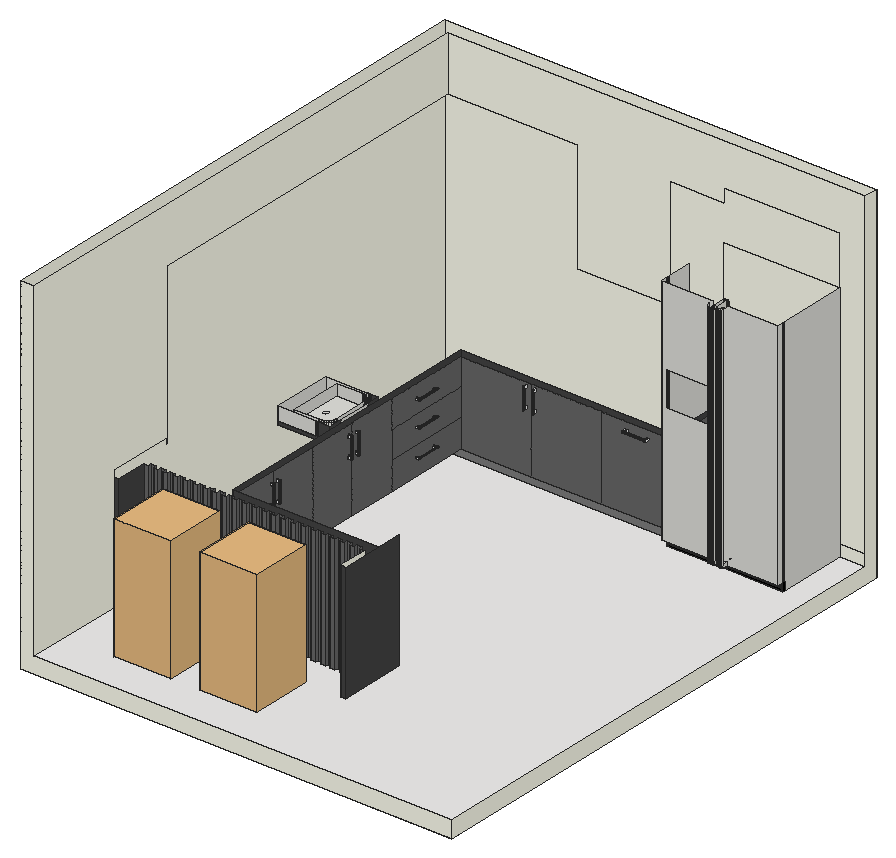
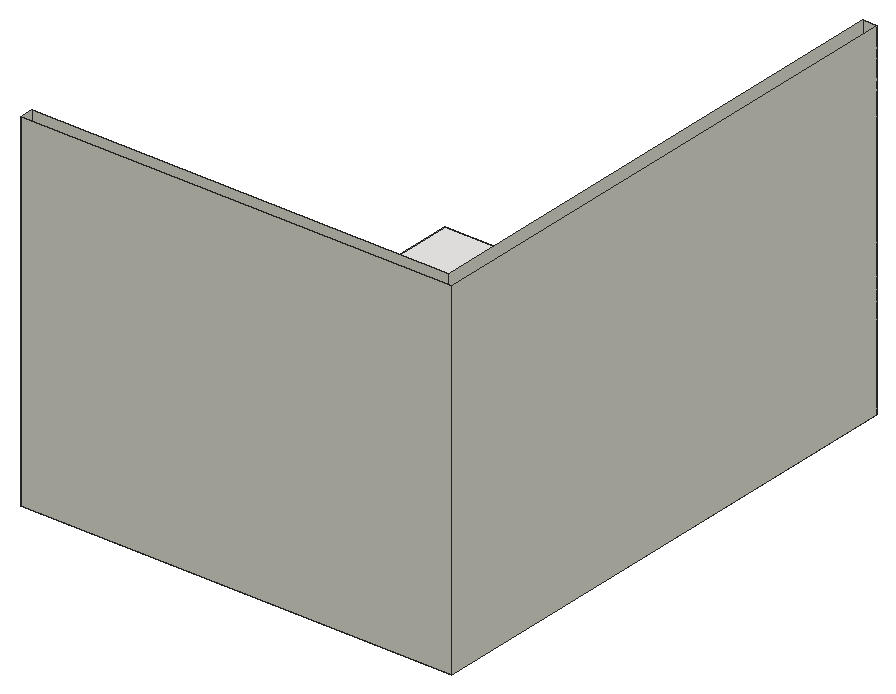
# SketchUp Ruby script. Lengths in inches.
U = 1.inch
M = Sketchup.active_model
def pt(a) = Geom::Point3d.new(a.map { |v| v * U })
def face(e, loops, mat)
  f = e.add_face(loops[0].map { |a| pt(a) })
  loops[1..].each { |l| e.add_face(l.map { |a| pt(a) }).erase! }
  f.material = f.back_material = mat if mat
  f
end
# faces: each face lists its corners as indices into pts; further lists are holes
def faces(e, pts, list, mat = nil) = list.each { |f| face(e, (f[0].is_a?(Array) ? f : [f]).map { |l| l.map { |i| pts[i] } }, mat) }
# xy, xz, yz: faces in a plane at the given z, y or x. An outline is a flat list of corners, or four numbers for a rectangle; further outlines are holes
def ring(l) = l.size == 4 ? [[l[0], l[1]], [l[2], l[1]], [l[2], l[3]], [l[0], l[3]]] : l.each_slice(2).to_a
def flat(e, list, mat, &to3) = list.each { |f| face(e, (f[0].is_a?(Array) ? f : [f]).map { |l| ring(l).map { |u, v| to3.(u, v) } }, mat) }
def xy(e, z, list, mat = nil) = flat(e, list, mat) { |x, y| [x, y, z] }
def xz(e, y, list, mat = nil) = flat(e, list, mat) { |x, z| [x, y, z] }
def yz(e, x, list, mat = nil) = flat(e, list, mat) { |y, z| [x, y, z] }
def lines(e, pts, list) = list.each { |a, b| e.add_line(pt(pts[a]), pt(pts[b])) }
# prism: a flat outline (further loops are holes) pulled along v
def prism(e, loops, v, mat = nil)
  f = face(e, loops, mat); d = Geom::Vector3d.new(v.map { |x| x * U })
  f.pushpull(f.normal.samedirection?(d) ? d.length : -d.length)
end
def box(e, o, s, mat = nil) = prism(e, [[o, [o[0] + s[0], o[1], o[2]], [o[0] + s[0], o[1] + s[1], o[2]], [o[0], o[1] + s[1], o[2]]]], [0, 0, s[2]], mat)
def at(x, y, z, deg = 0) = Geom::Transformation.translation(pt([x, y, z])) * Geom::Transformation.rotation(ORIGIN, Z_AXIS, deg.degrees)
def axes(o, x, y, z) = Geom::Transformation.new([*x, 0, *y, 0, *z, 0, *pt(o).to_a, 1])
def part(name) = M.definitions.add(name)
# library, detail: a bought-in or finely detailed component or shape, given as its bounding box
def library(name, o, s) = part(name).tap { |d| box(d.entities, o, s) }
def detail(e, o, s) = box(e.add_group.entities, o, s)
def put(e, d, t, mat = nil) = e.add_instance(d, t).tap { |i| i.material = mat if mat }
def group(e, t, mat = nil) = e.add_group.tap { |g| g.transformation = t; g.material = mat if mat }.entities
root = M.entities
M.materials.add("[0053_Ivory]").color = [255, 255, 240]
M.materials.add("[0128_White]").color = [255, 255, 255]
M.materials.add("[0133_Gray]").color = [128, 128, 128]
M.materials.add("[0134_DimGray]").color = [105, 105, 105]
M.materials.add("[0137_Black]").color = [0, 0, 0]
M.materials.add("[Granite Dark Gray]").color = [69, 68, 68]
M.materials.add("[Tile Limestone Large]").color = [241, 240, 239]
c1 = library("Group",[-8.82,-17.72,0],[17.64,35.44,18.29])
c2 = part("Bar")
prism(c2.entities,[[[0,0.49,0.31],[0,0.5,0.25],[0,0.49,0.19],[0,0.47,0.125],[0,0.43,0.07],[0,0.375,0.03],[0,0.31,0.01],[0,0.25,0],[0,0.19,0.01],[0,0.125,0.03],[0,0.07,0.07],[0,0.03,0.125],[0,0.01,0.19],[0,0,0.25],[0,0.01,0.31],[0,0.03,0.375],[0,0.07,0.43],[0,0.125,0.47],[0,0.19,0.49],[0,0.25,0.5],[0,0.31,0.49],[0,0.375,0.47],[0,0.43,0.43],[0,0.47,0.375]]],[11.5,0,0],"[0128_White]")
c3 = part("End")
xy(c3.entities,0,[[0,0.25,0.875,1.5]],"[0128_White]")
xy(c3.entities,0.5,[[0,0.25,0.875,1.5]],"[0128_White]")
xz(c3.entities,1.5,[[0,0,0.875,0.5]],"[0128_White]")
yz(c3.entities,0,[[0.25,0,0.19,0.01,0.125,0.03,0.07,0.07,0.03,0.125,0.01,0.19,0,0.25,0.01,0.31,0.03,0.375,0.07,0.43,0.125,0.47,0.19,0.49,0.25,0.5,1.5,0.5,1.5,0]],"[0128_White]")
yz(c3.entities,0.25,[[0.25,0,0.31,0.01,0.375,0.03,0.43,0.07,0.47,0.125,0.49,0.19,0.5,0.25,0.49,0.31,0.47,0.375,0.43,0.43,0.375,0.47,0.31,0.49,0.25,0.5,0.19,0.49,0.125,0.47,0.07,0.43,0.03,0.375,0.01,0.31,0,0.25,0.01,0.19,0.03,0.125,0.07,0.07,0.125,0.03,0.19,0.01]],"[0128_White]")
yz(c3.entities,0.875,[[0.25,0,1.5,0,1.5,0.5,0.25,0.5,0.31,0.49,0.375,0.47,0.43,0.43,0.47,0.375,0.49,0.31,0.5,0.25,0.49,0.19,0.47,0.125,0.43,0.07,0.375,0.03,0.31,0.01]],"[0128_White]")
p = [[0.25,0.125,0.03],[0,0.125,0.03],[0,0.19,0.01],[0.25,0.19,0.01],[0.25,0.07,0.07],[0,0.07,0.07],
  [0,0.25,0],[0.25,0.25,0],[0.875,0.25,0],[0.875,0.31,0.01],[0.25,0.31,0.01],[0.875,0.375,0.03],
  [0.25,0.375,0.03],[0.875,0.43,0.07],[0.25,0.43,0.07],[0.25,0.01,0.19],[0,0.01,0.19],[0,0.03,0.125],
  [0.25,0.03,0.125],[0.875,0.47,0.125],[0.25,0.47,0.125],[0.875,0.49,0.19],[0.25,0.49,0.19],[0.25,0.01,0.31],
  [0,0.01,0.31],[0,0,0.25],[0.25,0,0.25],[0.875,0.5,0.25],[0.25,0.5,0.25],[0.875,0.49,0.31],
  [0.25,0.49,0.31],[0.25,0.03,0.375],[0,0.03,0.375],[0.875,0.47,0.375],[0.25,0.47,0.375],[0.25,0.07,0.43],
  [0,0.07,0.43],[0.25,0.125,0.47],[0,0.125,0.47],[0.875,0.43,0.43],[0.25,0.43,0.43],[0.875,0.375,0.47],
  [0.25,0.375,0.47],[0.25,0.19,0.49],[0,0.19,0.49],[0.25,0.25,0.5],[0,0.25,0.5],[0.875,0.31,0.49],
  [0.875,0.25,0.5],[0.25,0.31,0.49]]
faces(c3.entities,p,[[0,1,2,3],[4,5,1,0],[3,2,6,7],[8,9,10,7],[9,11,12,10],[11,13,14,12],[15,16,17,18],[18,17,5,4],
  [13,19,20,14],[19,21,22,20],[23,24,25,26],[26,25,16,15],[21,27,28,22],[27,29,30,28],[31,32,24,23],[29,33,34,30],
  [35,36,32,31],[37,38,36,35],[33,39,40,34],[39,41,42,40],[43,44,38,37],[45,46,44,43],[47,48,45,49],[41,47,49,42]],"[0128_White]")
c4 = part("Drawer Pull\#1")
put(c4.entities,c2,axes([0.25,0,0],[0.71,0,0],[0,1,0],[0,0,1]))
put(c4.entities,c3,at(0,0,0))
put(c4.entities,c3,axes([8.66,0,0],[-1,0,0],[0,1,0],[0,0,1]),"[0128_White]")
c5 = part("Drawer Pull\#2")
put(c5.entities,c2,axes([0.25,0,0],[0.63,0,0],[0,1,0],[0,0,1]))
put(c5.entities,c3,at(0,0,0))
put(c5.entities,c3,axes([7.74,0,0],[-1,0,0],[0,1,0],[0,0,1]),"[0128_White]")
xy(root,0,[[0,0,156,192]],"[0053_Ivory]")
xy(root,6,[[104.87,161.36,125.37,161.36,125.37,161.85,126.37,161.85,126.37,161.36,146.87,161.36,146.87,187,104.87,187]])
xy(root,6,[[5,0,156,0,156,187,146.87,187,146.87,161.36,126.37,161.36,126.37,161.85,125.37,161.85,125.37,161.36,104.87,161.36,104.87,165,7,165,7,59.91,89,59.91,89,35.93,87,35.93,87,46.93,85.22,46.93,85.22,47.93,83.44,47.93,83.44,46.93,81.67,46.93,81.67,47.93,79.89,47.93,79.89,46.93,78.11,46.93,78.11,47.93,76.33,47.93,76.33,46.93,74.56,46.93,74.56,47.93,72.78,47.93,72.78,46.93,71,46.93,71,47.93,69.22,47.93,69.22,46.93,67.44,46.93,67.44,47.93,65.67,47.93,65.67,46.93,63.89,46.93,63.89,47.93,62.11,47.93,62.11,46.93,60.33,46.93,60.33,47.93,58.56,47.93,58.56,46.93,56.78,46.93,56.78,47.93,55,47.93,55,46.93,53.22,46.93,53.22,47.93,51.44,47.93,51.44,46.93,49.67,46.93,49.67,47.93,47.89,47.93,47.89,46.93,46.11,46.93,46.11,47.93,44.33,47.93,44.33,46.93,42.56,46.93,42.56,47.93,40.78,47.93,40.78,46.93,39,46.93,39,47.93,37.22,47.93,37.22,46.93,35.44,46.93,35.44,47.93,33.67,47.93,33.67,46.93,31.89,46.93,31.89,47.93,30.11,47.93,30.11,46.93,28.33,46.93,28.33,47.93,26.56,47.93,26.56,46.93,24.78,46.93,24.78,47.93,23,47.93,23,46.93,21.22,46.93,21.22,47.93,19.44,47.93,19.44,46.93,17.67,46.93,17.67,47.93,15.89,47.93,15.89,46.93,14.11,46.93,14.11,47.93,12.33,47.93,12.33,46.93,10.56,46.93,10.56,47.93,8.78,47.93,8.78,46.93,7,46.93,7,35.93,5,35.93]],"[Tile Limestone Large]")
xy(root,6.5,[[105.37,161.36,124.87,161.84],[126.87,161.36,146.37,161.85]],"[0137_Black]")
xy(root,7,[[105.87,161.36,124.37,161.84],[127.37,161.36,145.87,161.85]],"[0137_Black]")
xy(root,7.25,[[106.12,161.36,124.12,161.84],[127.62,161.36,145.62,161.85]],"[0137_Black]")
xy(root,7.74,[[106.12,161.36,124.12,161.84],[127.62,161.36,145.62,161.85]],"[0137_Black]")
xy(root,7.99,[[105.87,161.36,124.37,161.84],[127.37,161.36,145.87,161.85]],"[0137_Black]")
xy(root,8.49,[[105.37,161.36,124.87,161.84],[126.87,161.36,146.37,161.85]],"[0137_Black]")
xy(root,8.99,[[123.37,157.11,123.37,158.94,104.87,158.94,104.87,160.87,125.37,160.87,125.37,157.11],[126.37,157.11,126.37,160.88,146.87,160.88,146.87,158.94,128.37,158.94,128.37,157.11]])
xy(root,8.99,[[104.87,161.36,125.37,161.84],[126.37,161.36,146.87,161.85]],"[0137_Black]")
xy(root,9.99,[[123.37,157.01,125.37,158.94],[126.37,157.01,128.37,158.94]])
xy(root,10,[[7,59.91,29,165],[29,163,104.87,165]],"[0053_Ivory]")
xy(root,36,[[8.58,105.62,27.58,127.27]],"[Granite Dark Gray]")
xy(root,37.27,[[8.58,105.62,8.58,127.27,22.51,127.27,23.18,127.23,23.83,127.11,24.45,126.91,25.05,126.64,25.6,126.29,26.1,125.89,26.53,125.42,26.9,124.91,27.19,124.35,27.41,123.77,27.54,123.16,27.58,122.55,27.58,110.34,27.54,109.72,27.41,109.12,27.19,108.53,26.9,107.98,26.53,107.47,26.1,107,25.6,106.59,25.05,106.25,24.45,105.98,23.83,105.78,23.18,105.66,22.51,105.62]])
xy(root,38.0625,[[[13.65,106.8,22.47,106.8,23.01,106.83,23.5,106.92,23.97,107.07,24.41,107.27,24.83,107.53,25.2,107.84,25.53,108.1875,25.8,108.57,26.02,108.99,26.18,109.42,26.28,109.88,26.3125,110.38,26.3125,122.51,26.28,123.01,26.18,123.46,26.02,123.9,25.8,124.32,25.53,124.7,25.2,125.05,24.83,125.35,24.41,125.61,23.97,125.82,23.5,125.97,23.01,126.06,22.47,126.09,13.65,126.09],[17.45,115.66,17.23,115.68,17.03,115.76,16.85,115.89,16.72,116.05,16.64,116.24,16.61,116.44,16.64,116.65,16.72,116.84,16.85,117,17.03,117.125,17.23,117.2,17.45,117.23,17.67,117.2,17.87,117.125,18.05,117,18.18,116.84,18.27,116.65,18.3,116.44,18.27,116.24,18.18,116.05,18.05,115.89,17.87,115.76,17.67,115.68]],[17.45,115.66,17.67,115.68,17.87,115.76,18.05,115.89,18.18,116.05,18.27,116.24,18.3,116.44,18.27,116.65,18.18,116.84,18.05,117,17.87,117.125,17.67,117.2,17.45,117.23,17.23,117.2,17.03,117.125,16.85,117,16.72,116.84,16.64,116.65,16.61,116.44,16.64,116.24,16.72,116.05,16.85,115.89,17.03,115.76,17.23,115.68]])
xz(root,0,[[0,0,156,0,156,6,5,6,5,126,0,126]],"[0053_Ivory]")
xz(root,35.93,[[5,6,7,48.49],[87,6,89,48.49]],"[Granite Dark Gray]")
xz(root,46.93,[[7,6,8.78,48.49],[10.56,6,12.33,48.49],[14.11,6,15.89,48.49],[17.67,6,19.44,48.49],[21.22,6,23,48.49],
  [24.78,6,26.56,48.49],[28.33,6,30.11,48.49],[31.89,6,33.67,48.49],[35.44,6,37.22,48.49],[39,6,40.78,48.49],
  [42.56,6,44.33,48.49],[46.11,6,47.89,48.49],[49.67,6,51.44,48.49],[53.22,6,55,48.49],[56.78,6,58.56,48.49],
  [60.33,6,62.11,48.49],[63.89,6,65.67,48.49],[67.44,6,69.22,48.49],[71,6,72.78,48.49],[74.56,6,76.33,48.49],
  [78.11,6,79.89,48.49],[81.67,6,83.44,48.49],[85.22,6,87,48.49]],"[0134_DimGray]")
xz(root,47.93,[[8.78,6,10.56,48.49],[12.33,6,14.11,48.49],[15.89,6,17.67,48.49],[19.44,6,21.22,48.49],[23,6,24.78,48.49],
  [26.56,6,28.33,48.49],[30.11,6,31.89,48.49],[33.67,6,35.44,48.49],[37.22,6,39,48.49],[40.78,6,42.56,48.49],
  [44.33,6,46.11,48.49],[47.89,6,49.67,48.49],[51.44,6,53.22,48.49],[55,6,56.78,48.49],[58.56,6,60.33,48.49],
  [62.11,6,63.89,48.49],[65.67,6,67.44,48.49],[69.22,6,71,48.49],[72.78,6,74.56,48.49],[76.33,6,78.11,48.49],
  [79.89,6,81.67,48.49],[83.44,6,85.22,48.49]],"[0134_DimGray]")
xz(root,59.91,[[7,6,7,10,29,10,29,42,89,42,89,6]],"[Granite Dark Gray]")
xz(root,105.62,[[8.58,37.27,22.51,42]])
xz(root,105.62,[[8.58,36,8.58,37.27,22.51,37.27,22.51,42,27.58,42,27.58,36]],"[Granite Dark Gray]")
xz(root,106.8,[[13.65,38.0625,22.47,42]])
xz(root,126.09,[[13.65,38.0625,22.47,42]])
xz(root,127.27,[[8.58,37.27,22.51,42]])
xz(root,127.27,[[8.58,36,27.58,36,27.58,42,22.51,42,22.51,37.27,8.58,37.27]],"[Granite Dark Gray]")
xz(root,157.01,[[123.37,9.99,125.37,91.99],[126.37,9.99,128.37,91.99]])
xz(root,158.94,[[[104.87,8.99,123.37,8.99,123.37,9.99,125.37,9.99,125.37,91.99,123.37,91.99,123.37,92.99,104.87,92.99],[106.25,52.26,122.66,64.76]],[128.37,8.99,146.87,8.99,146.87,92.99,128.37,92.99,128.37,91.99,126.37,91.99,126.37,9.99,128.37,9.99]])
xz(root,161.36,[[[104.87,6,125.37,8.99],[105.37,6.5,124.87,8.49]],[[126.37,6,146.87,8.99],[126.87,6.5,146.37,8.49]],[[105.87,7,124.37,7.99],[106.12,7.25,124.12,7.74]],[[127.37,7,145.87,7.99],[127.62,7.25,145.62,7.74]]],"[0137_Black]")
xz(root,161.84,[[[105.37,6.5,124.87,8.49],[105.87,7,124.37,7.99]],[106.12,7.25,124.12,7.74]],"[0134_DimGray]")
xz(root,161.85,[[125.37,6,125.87,92.99],[125.87,6,126.37,92.99]])
xz(root,161.85,[[[126.87,6.5,146.37,8.49],[127.37,7,145.87,7.99]],[127.62,7.25,145.62,7.74]],"[0134_DimGray]")
xz(root,163,[[29,10,54.29,40],[54.29,10,79.58,40],[79.58,10,104.87,40]],"[0134_DimGray]")
xz(root,163,[[29,40,104.87,42]],"[Granite Dark Gray]")
xz(root,165,[[7,6,104.87,10]],"[0133_Gray]")
xz(root,187,[[104.87,6,146.87,10],[146.87,6,156,10],[146.87,10,156,10,156,126,5,126,5,106,52,106,52,66,85.34,66,85.34,106,104.87,106,104.87,110.79,146.87,110.79],[104.87,10,146.87,92.99]],"[0053_Ivory]")
xz(root,192,[[0,0,156,126]],"[0053_Ivory]")
yz(root,0,[[0,0,192,126]],"[0053_Ivory]")
yz(root,5,[[0,6,35.93,6,35.93,50.49,59.93,50.49,59.93,48.49,60,66,60,106,187,106,187,126,0,126]],"[0053_Ivory]")
yz(root,7,[[59.91,6,165,10]],"[0133_Gray]")
yz(root,7,[[35.93,6,46.93,48.49]],"[Granite Dark Gray]")
yz(root,8.58,[[105.62,37.27,127.27,42]])
yz(root,8.58,[[105.62,36,127.27,37.27]],"[Granite Dark Gray]")
yz(root,8.78,[[46.93,6,47.93,48.49]],"[0134_DimGray]")
yz(root,10.56,[[46.93,6,47.93,48.49]],"[0134_DimGray]")
yz(root,12.33,[[46.93,6,47.93,48.49]],"[0134_DimGray]")
yz(root,13.65,[[106.8,38.0625,126.09,42]])
yz(root,14.11,[[46.93,6,47.93,48.49]],"[0134_DimGray]")
yz(root,15.89,[[46.93,6,47.93,48.49]],"[0134_DimGray]")
yz(root,17.67,[[46.93,6,47.93,48.49]],"[0134_DimGray]")
yz(root,19.44,[[46.93,6,47.93,48.49]],"[0134_DimGray]")
yz(root,21.22,[[46.93,6,47.93,48.49]],"[0134_DimGray]")
yz(root,23,[[46.93,6,47.93,48.49]],"[0134_DimGray]")
yz(root,24.78,[[46.93,6,47.93,48.49]],"[0134_DimGray]")
yz(root,26.3125,[[110.38,38.0625,122.51,42]])
yz(root,26.56,[[46.93,6,47.93,48.49]],"[0134_DimGray]")
yz(root,27.58,[[110.34,37.27,122.55,42]])
yz(root,27.58,[[105.62,36,105.62,42,110.34,42,110.34,37.27,122.55,37.27,122.55,42,127.27,42,127.27,36]],"[Granite Dark Gray]")
yz(root,28.33,[[46.93,6,47.93,48.49]],"[0134_DimGray]")
yz(root,29,[[59.91,10,77.91,40],[77.91,10,95.8125,40],[95.8125,10,113.72,40],[113.72,10,131.625,40],[131.625,10,163,20],
  [131.625,20,163,30],[131.625,30,163,40]],"[0134_DimGray]")
yz(root,29,[[59.91,40,163,42]],"[Granite Dark Gray]")
yz(root,30.11,[[46.93,6,47.93,48.49]],"[0134_DimGray]")
yz(root,31.89,[[46.93,6,47.93,48.49]],"[0134_DimGray]")
yz(root,33.67,[[46.93,6,47.93,48.49]],"[0134_DimGray]")
yz(root,35.44,[[46.93,6,47.93,48.49]],"[0134_DimGray]")
yz(root,37.22,[[46.93,6,47.93,48.49]],"[0134_DimGray]")
yz(root,39,[[46.93,6,47.93,48.49]],"[0134_DimGray]")
yz(root,40.78,[[46.93,6,47.93,48.49]],"[0134_DimGray]")
yz(root,42.56,[[46.93,6,47.93,48.49]],"[0134_DimGray]")
yz(root,44.33,[[46.93,6,47.93,48.49]],"[0134_DimGray]")
yz(root,46.11,[[46.93,6,47.93,48.49]],"[0134_DimGray]")
yz(root,47.89,[[46.93,6,47.93,48.49]],"[0134_DimGray]")
yz(root,49.67,[[46.93,6,47.93,48.49]],"[0134_DimGray]")
yz(root,51.44,[[46.93,6,47.93,48.49]],"[0134_DimGray]")
yz(root,53.22,[[46.93,6,47.93,48.49]],"[0134_DimGray]")
yz(root,55,[[46.93,6,47.93,48.49]],"[0134_DimGray]")
yz(root,56.78,[[46.93,6,47.93,48.49]],"[0134_DimGray]")
yz(root,58.56,[[46.93,6,47.93,48.49]],"[0134_DimGray]")
yz(root,60.33,[[46.93,6,47.93,48.49]],"[0134_DimGray]")
yz(root,62.11,[[46.93,6,47.93,48.49]],"[0134_DimGray]")
yz(root,63.89,[[46.93,6,47.93,48.49]],"[0134_DimGray]")
yz(root,65.67,[[46.93,6,47.93,48.49]],"[0134_DimGray]")
yz(root,67.44,[[46.93,6,47.93,48.49]],"[0134_DimGray]")
yz(root,69.22,[[46.93,6,47.93,48.49]],"[0134_DimGray]")
yz(root,71,[[46.93,6,47.93,48.49]],"[0134_DimGray]")
yz(root,72.78,[[46.93,6,47.93,48.49]],"[0134_DimGray]")
yz(root,74.56,[[46.93,6,47.93,48.49]],"[0134_DimGray]")
yz(root,76.33,[[46.93,6,47.93,48.49]],"[0134_DimGray]")
yz(root,78.11,[[46.93,6,47.93,48.49]],"[0134_DimGray]")
yz(root,79.89,[[46.93,6,47.93,48.49]],"[0134_DimGray]")
yz(root,81.67,[[46.93,6,47.93,48.49]],"[0134_DimGray]")
yz(root,83.44,[[46.93,6,47.93,48.49]],"[0134_DimGray]")
yz(root,85.22,[[46.93,6,47.93,48.49]],"[0134_DimGray]")
yz(root,87,[[35.93,6,46.93,48.49]],"[0053_Ivory]")
yz(root,89,[[35.93,6,59.91,6,59.91,42,59.93,48.49,35.93,48.49]],"[Granite Dark Gray]")
yz(root,104.87,[[161.84,6,161.84,92.99,171,92.99,171,66,185,66,185,42,163,42,163,10,165,10,165,6],[158.94,8.99,160.87,92.99]])
yz(root,104.87,[[165,6,187,10]],"[0133_Gray]")
yz(root,104.87,[[163,10,187,40]],"[0134_DimGray]")
yz(root,104.87,[[161.36,6,161.84,8.99]],"[0137_Black]")
yz(root,104.87,[[163,40,187,42]],"[Granite Dark Gray]")
yz(root,105.37,[[161.36,6.5,161.84,8.49]],"[0137_Black]")
yz(root,105.87,[[161.36,7,161.84,7.99]],"[0137_Black]")
yz(root,106.12,[[161.36,7.25,161.84,7.74]],"[0137_Black]")
yz(root,123.37,[[157.11,8.99,158.94,9.99]])
yz(root,124.12,[[161.36,7.25,161.84,7.74]],"[0137_Black]")
yz(root,124.37,[[161.36,7,161.84,7.99]],"[0137_Black]")
yz(root,124.87,[[161.36,6.5,161.84,8.49]],"[0137_Black]")
yz(root,125.37,[[157.11,8.99,160.87,8.99,160.87,92.99,157.11,92.99,157.11,91.99,158.94,91.99,158.94,9.99,157.11,9.99]])
yz(root,125.37,[[161.36,6,161.85,6,161.85,92.99,161.84,92.99,161.84,8.99,161.36,8.99]],"[0137_Black]")
yz(root,126.37,[[157.11,8.99,157.11,9.99,158.94,9.99,158.94,91.99,157.11,91.99,157.11,92.99,160.88,92.99,160.88,8.99]])
yz(root,126.37,[[161.36,6,161.85,8.99]],"[0137_Black]")
yz(root,126.87,[[161.36,6.5,161.85,8.49]],"[0137_Black]")
yz(root,127.37,[[161.36,7,161.85,7.99]],"[0137_Black]")
yz(root,127.62,[[161.36,7.25,161.85,7.74]],"[0137_Black]")
yz(root,128.37,[[157.11,8.99,158.94,9.99]])
yz(root,145.62,[[161.36,7.25,161.85,7.74]],"[0137_Black]")
yz(root,145.87,[[161.36,7,161.85,7.99]],"[0137_Black]")
yz(root,146.37,[[161.36,6.5,161.85,8.49]],"[0137_Black]")
yz(root,146.87,[[161.85,6,187,92.99],[158.94,8.99,160.88,92.99]])
yz(root,146.87,[[161.36,6,161.85,8.99]],"[0137_Black]")
yz(root,156,[[0,0,192,0,192,126,187,126,187,6,0,6]],"[0053_Ivory]")
p = [[123.5,156.62,9.13],[123.4,156.86,9.03],[125.33,156.86,9.03],[125.23,156.62,9.13],[123.5,156.62,92.86],[123.4,156.86,92.96],
  [123.4,156.86,91.03],[123.4,156.86,10.96],[123.5,156.62,10.86],[123.5,156.62,91.13],[125.33,156.86,10.96],[125.33,156.86,91.03],
  [125.33,156.86,92.96],[125.23,156.62,92.86],[125.23,156.62,91.13],[125.23,156.62,10.86],[128.33,156.86,9.03],[128.23,156.62,9.13],
  [126.5,156.62,9.13],[126.4,156.86,9.03],[126.5,156.62,10.86],[126.5,156.62,91.13],[126.5,156.62,92.86],[126.4,156.86,92.96],
  [126.4,156.86,91.03],[126.4,156.86,10.96],[128.33,156.86,92.96],[128.23,156.62,92.86],[128.23,156.62,91.13],[128.23,156.62,10.86],
  [128.33,156.86,10.96],[128.33,156.86,91.03],[123.37,157.11,8.99],[125.37,157.11,8.99],[123.37,157.11,92.99],[123.37,157.11,91.99],
  [123.37,157.11,90.99],[123.37,157.11,10.99],[123.37,157.11,9.99],[125.37,157.11,9.99],[125.37,157.11,10.99],[125.37,157.11,90.99],
  [125.37,157.11,91.99],[125.37,157.11,92.99],[128.37,157.11,8.99],[126.37,157.11,8.99],[126.37,157.11,92.99],[126.37,157.11,91.99],
  [126.37,157.11,90.99],[126.37,157.11,10.99],[126.37,157.11,9.99],[128.37,157.11,92.99],[128.37,157.11,9.99],[128.37,157.11,10.99],
  [128.37,157.11,90.99],[128.37,157.11,91.99],[125.24,160.89,9.125],[125.37,160.87,8.99],[104.87,160.87,8.99],[105,160.89,9.125],
  [104.87,160.87,92.99],[105,160.89,92.86],[125.24,160.89,92.86],[125.37,160.87,92.99],[146.74,160.89,9.125],[146.87,160.88,8.99],
  [126.37,160.88,8.99],[126.5,160.89,9.125],[126.37,160.88,92.99],[126.5,160.89,92.86],[146.74,160.89,92.86],[146.87,160.88,92.99],
  [125.37,161.84,8.99],[125.24,161.83,9.125],[105,161.83,9.125],[104.87,161.84,8.99],[105,161.83,92.86],[104.87,161.84,92.99],
  [125.37,161.84,92.99],[125.24,161.83,92.86],[146.87,161.85,8.99],[146.74,161.83,9.125],[126.5,161.83,9.125],[126.37,161.85,8.99],
  [126.5,161.83,92.86],[126.37,161.85,92.99],[146.87,161.85,92.99],[146.74,161.83,92.86],[123.66,156.42,9.29],[125.07,156.42,9.29],
  [123.66,156.42,92.7],[123.66,156.42,10.7],[123.66,156.42,91.29],[125.07,156.42,92.7],[125.07,156.42,91.29],[125.07,156.42,10.7],
  [128.07,156.42,9.29],[126.66,156.42,9.29],[126.66,156.42,10.7],[126.66,156.42,91.29],[126.66,156.42,92.7],[128.07,156.42,92.7],
  [128.07,156.42,91.29],[128.07,156.42,10.7],[125.11,160.9375,9.24],[105.12,160.9375,9.24],[105.12,160.9375,92.74],[125.11,160.9375,92.74],
  [146.62,160.94,9.24],[126.62,160.94,9.24],[126.62,160.94,92.74],[146.62,160.94,92.74],[125.11,161.78,9.24],[105.12,161.78,9.24],
  [105.12,161.78,92.74],[125.11,161.78,92.74],[146.62,161.78,9.24],[126.62,161.78,9.24],[126.62,161.78,92.74],[146.62,161.78,92.74],
  [125.01,161.01,9.35],[105.22,161.01,9.35],[105.22,161.01,92.64],[125.01,161.01,92.64],[146.51,161.02,9.35],[126.72,161.02,9.35],
  [126.72,161.02,92.64],[146.51,161.02,92.64],[125.01,161.7,9.35],[105.22,161.7,9.35],[105.22,161.7,92.64],[125.01,161.7,92.64],
  [146.51,161.7,9.35],[126.72,161.7,9.35],[126.72,161.7,92.64],[146.51,161.7,92.64],[123.87,156.27,9.49],[124.87,156.27,9.49],
  [123.87,156.27,92.49],[123.87,156.27,10.49],[123.87,156.27,91.49],[124.87,156.27,92.49],[124.87,156.27,91.49],[124.87,156.27,10.49],
  [127.87,156.27,9.49],[126.87,156.27,9.49],[126.87,156.27,10.49],[126.87,156.27,91.49],[126.87,156.27,92.49],[127.87,156.27,92.49],
  [127.87,156.27,91.49],[127.87,156.27,10.49],[124.93,161.11,9.43],[105.3,161.11,9.43],[105.3,161.11,92.56],[124.93,161.11,92.56],
  [146.43,161.12,9.43],[126.8,161.12,9.43],[126.8,161.12,92.5625],[146.43,161.12,92.5625],[124.93,161.6,9.43],[105.3,161.6,9.43],
  [105.3,161.6,92.56],[124.93,161.6,92.56],[146.43,161.6,9.43],[126.8,161.6,9.43],[126.8,161.6,92.5625],[146.43,161.6,92.5625],
  [124.88,161.23,9.48],[105.35,161.23,9.48],[105.35,161.23,92.51],[124.88,161.23,92.51],[146.38,161.24,9.48],[126.85,161.24,9.48],
  [126.85,161.24,92.51],[146.38,161.24,92.51],[124.88,161.48,9.48],[105.35,161.48,9.48],[105.35,161.48,92.51],[124.88,161.48,92.51],
  [146.38,161.49,9.48],[126.85,161.49,9.48],[126.85,161.49,92.51],[146.38,161.49,92.51],[124.11,156.17,9.74],[124.625,156.17,9.74],
  [124.11,156.17,92.25],[124.11,156.17,10.25],[124.11,156.17,91.74],[124.625,156.17,92.25],[124.625,156.17,91.74],[124.625,156.17,10.25],
  [127.625,156.17,9.74],[127.11,156.17,9.74],[127.11,156.17,10.25],[127.11,156.17,91.74],[127.11,156.17,92.25],[127.625,156.17,92.25],
  [127.625,156.17,91.74],[127.625,156.17,10.25],[124.86,161.36,9.5],[105.37,161.36,9.5],[105.37,161.36,92.49],[124.86,161.36,92.49],
  [146.37,161.36,9.49],[126.87,161.36,9.49],[126.87,161.36,92.49],[146.37,161.36,92.49],[124.37,156.14,9.99],[124.37,156.14,91.99],
  [127.37,156.14,9.99],[127.37,156.14,91.99],[23.18,105.66,37.27],[23.18,105.66,42],[22.51,105.62,42],[22.51,105.62,37.27],
  [23.83,105.78,37.27],[23.83,105.78,42],[24.45,105.98,37.27],[24.45,105.98,42],[25.05,106.25,37.27],[25.05,106.25,42],
  [25.6,106.59,37.27],[25.6,106.59,42],[26.1,107,37.27],[26.1,107,42],[26.53,107.47,37.27],[26.53,107.47,42],
  [26.9,107.98,37.27],[26.9,107.98,42],[27.19,108.53,37.27],[27.19,108.53,42],[27.41,109.12,37.27],[27.41,109.12,42],
  [27.54,109.72,37.27],[27.54,109.72,42],[27.58,110.34,37.27],[27.58,110.34,42],[27.58,122.55,37.27],[27.54,123.16,37.27],
  [27.54,123.16,42],[27.58,122.55,42],[27.41,123.77,37.27],[27.41,123.77,42],[27.19,124.35,37.27],[27.19,124.35,42],
  [26.9,124.91,37.27],[26.9,124.91,42],[26.53,125.42,37.27],[26.53,125.42,42],[26.1,125.89,37.27],[26.1,125.89,42],
  [25.6,126.29,37.27],[25.6,126.29,42],[25.05,126.64,37.27],[25.05,126.64,42],[24.45,126.91,37.27],[24.45,126.91,42],
  [23.83,127.11,37.27],[23.83,127.11,42],[23.18,127.23,37.27],[23.18,127.23,42],[22.51,127.27,37.27],[22.51,127.27,42],
  [22.47,106.8,38.0625],[22.47,106.8,42],[23.01,106.83,42],[23.01,106.83,38.0625],[23.5,106.92,42],[23.5,106.92,38.0625],
  [23.97,107.07,42],[23.97,107.07,38.0625],[24.41,107.27,42],[24.41,107.27,38.0625],[24.83,107.53,42],[24.83,107.53,38.0625],
  [25.2,107.84,42],[25.2,107.84,38.0625],[25.53,108.1875,42],[25.53,108.1875,38.0625],[25.8,108.57,42],[25.8,108.57,38.0625],
  [26.02,108.99,42],[26.02,108.99,38.0625],[26.18,109.42,42],[26.18,109.42,38.0625],[26.28,109.88,42],[26.28,109.88,38.0625],
  [26.3125,110.38,42],[26.3125,110.38,38.0625],[26.3125,122.51,42],[26.28,123.01,42],[26.28,123.01,38.0625],[26.3125,122.51,38.0625],
  [26.18,123.46,42],[26.18,123.46,38.0625],[26.02,123.9,42],[26.02,123.9,38.0625],[25.8,124.32,42],[25.8,124.32,38.0625],
  [25.53,124.7,42],[25.53,124.7,38.0625],[25.2,125.05,42],[25.2,125.05,38.0625],[24.83,125.35,42],[24.83,125.35,38.0625],
  [24.41,125.61,42],[24.41,125.61,38.0625],[23.97,125.82,42],[23.97,125.82,38.0625],[23.5,125.97,42],[23.5,125.97,38.0625],
  [23.01,126.06,42],[23.01,126.06,38.0625],[22.47,126.09,42],[22.47,126.09,38.0625],[24.52,34.61,5.71],[23.35,34.61,5.71],
  [23.35,33.4,5.71],[55.45,34.61,5.71],[54.29,34.61,5.71],[54.29,33.4,5.71],[29,163,40],[29,165,40]]
faces(root,p,[[0,1,2,3],[4,5,6,7,1,0,8,9],[3,2,10,11,12,13,14,15],[16,17,18,19],[19,18,20,21,22,23,24,25],[26,27,28,29,17,16,30,31],[1,32,33,2],[5,34,35,36,37,38,32,1,7,6],
  [2,33,39,40,41,42,43,12,11,10],[44,16,19,45],[45,19,25,24,23,46,47,48,49,50],[51,26,31,30,16,44,52,53,54,55],[88,0,3,89],[90,4,9,8,0,88,91,92],[89,3,15,14,13,93,94,95],[17,96,97,18],
  [18,97,98,99,100,22,21,20],[27,101,102,103,96,17,29,28],[136,88,89,137],[138,90,92,91,88,136,139,140],[137,89,95,94,93,141,142,143],[96,144,145,97],[97,145,146,147,148,100,99,98],[101,149,150,151,144,96,103,102],
  [184,136,137,185],[186,138,140,139,136,184,187,188],[185,137,143,142,141,189,190,191],[144,192,193,145],[145,193,194,195,196,148,147,146],[149,197,198,199,192,144,151,150],[208,184,185],[209,186,188,187,184,208],
  [208,185,191,190,189,209],[192,210,193],[193,210,211,196,195,194],[197,211,210,192,199,198],[212,213,214,215],[216,217,213,212],[218,219,217,216],[220,221,219,218],
  [222,223,221,220],[224,225,223,222],[224,226,227,225],[226,228,229,227],[228,230,231,229],[230,232,233,231],[232,234,235,233],[234,236,237,235],
  [238,239,240,241],[239,242,243,240],[242,244,245,243],[244,246,247,245],[246,248,249,247],[248,250,251,249],[252,253,251,250],[254,255,253,252],
  [256,257,255,254],[258,259,257,256],[260,261,259,258],[262,263,261,260],[264,265,266,267],[267,266,268,269],[269,268,270,271],[271,270,272,273],
  [273,272,274,275],[275,274,276,277],[276,278,279,277],[278,280,281,279],[280,282,283,281],[282,284,285,283],[284,286,287,285],[286,288,289,287],
  [290,291,292,293],[291,294,295,292],[294,296,297,295],[296,298,299,297],[298,300,301,299],[300,302,303,301],[303,302,304,305],[305,304,306,307],
  [307,306,308,309],[309,308,310,311],[311,310,312,313],[313,312,314,315]])
faces(root,p,[[56,57,58,59],[59,58,60,61],[62,63,57,56],[64,65,66,67],[67,66,68,69],[70,71,65,64],[72,73,74,75],[75,74,76,77],
  [78,79,73,72],[80,81,82,83],[83,82,84,85],[86,87,81,80],[104,56,59,105],[105,59,61,106],[107,62,56,104],[108,64,67,109],
  [109,67,69,110],[111,70,64,108],[73,112,113,74],[74,113,114,76],[79,115,112,73],[81,116,117,82],[82,117,118,84],[87,119,116,81],
  [120,104,105,121],[121,105,106,122],[123,107,104,120],[124,108,109,125],[125,109,110,126],[127,111,108,124],[112,128,129,113],[113,129,130,114],
  [115,131,128,112],[116,132,133,117],[117,133,134,118],[119,135,132,116],[152,120,121,153],[153,121,122,154],[155,123,120,152],[156,124,125,157],
  [157,125,126,158],[159,127,124,156],[128,160,161,129],[129,161,162,130],[131,163,160,128],[132,164,165,133],[133,165,166,134],[135,167,164,132],
  [168,152,153,169],[169,153,154,170],[171,155,152,168],[172,156,157,173],[173,157,158,174],[175,159,156,172],[160,176,177,161],[161,177,178,162],
  [163,179,176,160],[164,180,181,165],[165,181,182,166],[167,183,180,164],[200,168,169,201],[201,169,170,202],[203,171,168,200],[204,172,173,205],
  [205,173,174,206],[207,175,172,204],[176,200,201,177],[177,201,202,178],[179,203,200,176],[180,204,205,181],[181,205,206,182],[183,207,204,180]],"[0137_Black]")
lines(root,p,[[316,317],[317,318],[318,316],[319,320],[320,321],[321,319],[322,323]])
put(root,c1,axes([32.87,14.2,28.1],[-1.16557,0,0],[0,0,1.26363],[0,1.21,0]))
put(root,c1,axes([63.8,14.2,28.1],[-1.16557,0,0],[0,0,1.26363],[0,1.21,0]))
put(root,c4,at(30.5,142.22,16.17,90),"[0128_White]")
put(root,c4,at(30.5,142.22,25.98,90),"[0128_White]")
put(root,c5,axes([30.5,111.67,37.19],[0,0,-1],[-1,0,0],[0,1,0]),"[0128_White]")
put(root,c5,axes([30.5,114.98,37.19],[0,0,-1],[-1,0,0],[0,1,0]),"[0128_White]")
put(root,c5,axes([30.5,79.17,37.19],[0,0,-1],[-1,0,0],[0,1,0]),"[0128_White]")
put(root,c5,axes([30.5,76.48,37.19],[0,0,-1],[-1,0,0],[0,1,0]),"[0128_White]")
put(root,c5,axes([55.71,161.5,39.1],[0,0,-1],[0,1,0],[1,0,0]),"[0128_White]")
put(root,c5,axes([52.33,161.5,39.1],[0,0,-1],[0,1,0],[1,0,0]),"[0128_White]")
put(root,c4,at(30.5,142.22,35.11,90),"[0128_White]")
put(root,c4,at(88.36,161.5,36.8),"[0128_White]")
